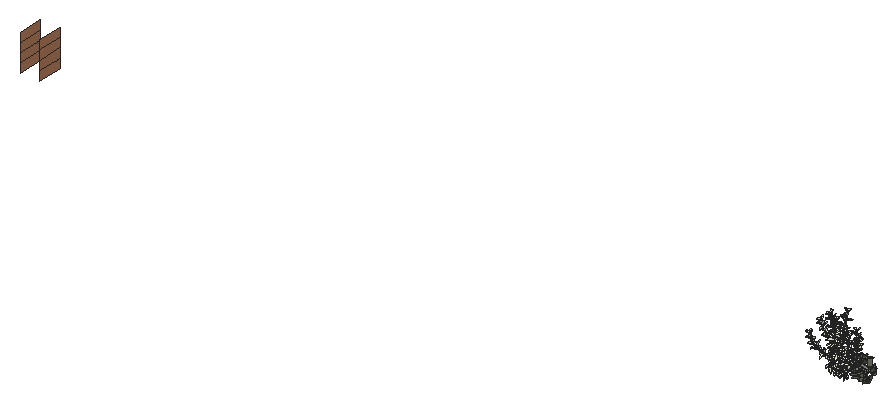
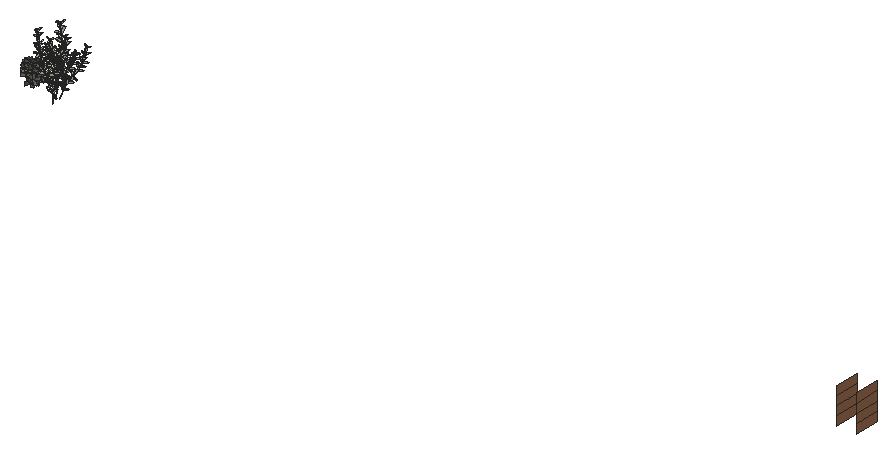
# SketchUp Ruby script. Lengths in inches.
U = 1.inch
M = Sketchup.active_model
def pt(a) = Geom::Point3d.new(a.map { |v| v * U })
def face(e, loops, mat)
  f = e.add_face(loops[0].map { |a| pt(a) })
  loops[1..].each { |l| e.add_face(l.map { |a| pt(a) }).erase! }
  f.material = f.back_material = mat if mat
  f
end
# faces: each face lists its corners as indices into pts; further lists are holes
def faces(e, pts, list, mat = nil) = list.each { |f| face(e, (f[0].is_a?(Array) ? f : [f]).map { |l| l.map { |i| pts[i] } }, mat) }
# xy, xz, yz: faces in a plane at the given z, y or x. An outline is a flat list of corners, or four numbers for a rectangle; further outlines are holes
def ring(l) = l.size == 4 ? [[l[0], l[1]], [l[2], l[1]], [l[2], l[3]], [l[0], l[3]]] : l.each_slice(2).to_a
def flat(e, list, mat, &to3) = list.each { |f| face(e, (f[0].is_a?(Array) ? f : [f]).map { |l| ring(l).map { |u, v| to3.(u, v) } }, mat) }
def xy(e, z, list, mat = nil) = flat(e, list, mat) { |x, y| [x, y, z] }
def xz(e, y, list, mat = nil) = flat(e, list, mat) { |x, z| [x, y, z] }
def yz(e, x, list, mat = nil) = flat(e, list, mat) { |y, z| [x, y, z] }
def lines(e, pts, list) = list.each { |a, b| e.add_line(pt(pts[a]), pt(pts[b])) }
# prism: a flat outline (further loops are holes) pulled along v
def prism(e, loops, v, mat = nil)
  f = face(e, loops, mat); d = Geom::Vector3d.new(v.map { |x| x * U })
  f.pushpull(f.normal.samedirection?(d) ? d.length : -d.length)
end
def box(e, o, s, mat = nil) = prism(e, [[o, [o[0] + s[0], o[1], o[2]], [o[0] + s[0], o[1] + s[1], o[2]], [o[0], o[1] + s[1], o[2]]]], [0, 0, s[2]], mat)
def at(x, y, z, deg = 0) = Geom::Transformation.translation(pt([x, y, z])) * Geom::Transformation.rotation(ORIGIN, Z_AXIS, deg.degrees)
def axes(o, x, y, z) = Geom::Transformation.new([*x, 0, *y, 0, *z, 0, *pt(o).to_a, 1])
def part(name) = M.definitions.add(name)
# library, detail: a bought-in or finely detailed component or shape, given as its bounding box
def library(name, o, s) = part(name).tap { |d| box(d.entities, o, s) }
def detail(e, o, s) = box(e.add_group.entities, o, s)
def put(e, d, t, mat = nil) = e.add_instance(d, t).tap { |i| i.material = mat if mat }
def group(e, t, mat = nil) = e.add_group.tap { |g| g.transformation = t; g.material = mat if mat }.entities
root = M.entities
M.materials.add("0ad16as01f6asdLeafVar1sfd015as60f1as6").color = [231, 235, 211]
M.materials.add("[Tile Ceramic Multi]").color = [165, 115, 84]
M.materials.add("asdfasdf0165f6asdLeafVar1sfd015as60f1as6").color = [231, 235, 211]
M.materials.add("dw_stemssadfasdfa0sdf1s01d6w1").color = [90, 97, 50]
M.materials.add("viburnumblaasdfas0df1w06d").color = [98, 102, 84]
M.materials.add("viburnumbladsadfasdfad0w122").color = [125, 129, 119]
c1 = part("Component\#315")
p = [[0.25,0,0],[2.05,0.01,0.35],[1.81,4.2,1.66],[0,4.19,1.3125]]
faces(c1.entities,p,[[0,1,2,3]],"viburnumbladsadfasdfad0w122")
c2 = part("viburnumblad2")
put(c2.entities,c1,axes([-19.23,-4.49,-32.18],[83.35428,0,0],[0,79.38502,0],[0,0,83.35428]))
c3 = part("Component\#314")
p = [[0.14,0,0],[2.58,0.05,0.25],[2.44,5.11,2.64],[0,5.05,2.39]]
faces(c3.entities,p,[[0,1,2,3]],"viburnumblaasdfas0df1w06d")
c4 = part("viburnumblad1\#2")
put(c4.entities,c3,axes([-37.25,6.23,19.31],[75.98784,0,0],[0,65.50676,0],[0,0,75.98784]))
c5 = part("vdw_leaf\#1")
p = [[0,0,0],[-2.77,1.61,2.32],[-4.3125,6.1,4.5],[-3.97,13.49,6.09],[-2.47,18.57,6.3],[-0.2,22.73,5.75],
  [2.54,19.66,6.85],[4.3,15.93,7.09],[5.03,7.6,5.43],[3.32,1.76,2.74]]
faces(c5.entities,p,[[0,1,2,3,4,5],[0,5,6,7,8,9]],"0ad16as01f6asdLeafVar1sfd015as60f1as6")
c6 = part("dw_branch_3\#2")
p = [[-10.06,-1.6,62.9],[-0.2,1.54,-0.01],[-10.43,1.54,62.72],[0.18,-1.6,0.17],[-23.75,-21.66,88.91],[-25.7,-20.3,89.55],
  [13.4,11.62,104.56],[13.33,13.52,104.47],[-49.25,-41.87,130.3125],[-50.33,-40.21,130.71],[-4.97,21.13,143.98],[35.61,27.99,178.64],
  [-5.09,23.64,143.96],[35.32,29.14,178.46],[-67.7,-55.38,181.06],[-68.34,-54.45,181.62],[-22.8125,33.9,200.59],[-22.94,35.79,200.41],
  [56.61,36.78,229.75],[56.29,38.09,229.57],[-70.63,-67.46,248.85],[-70.72,-66.33,249.5],[-25.05,43.32,240.75],[-24.98,44.26,240.57]]
faces(c6.entities,p,[[0,1,2],[0,3,1],[4,2,5],[4,0,2],[6,0,2],[6,2,7],[8,4,5],[8,5,9],
  [10,6,7],[11,6,7],[10,7,12],[11,7,13],[14,8,9],[14,9,15],[16,10,12],[16,12,17],
  [18,11,13],[18,13,19],[20,14,15],[20,15,21],[22,16,17],[22,17,23]],"dw_stemssadfasdfa0sdf1s01d6w1")
c7 = part("dw_branch3\#2")
put(c7.entities,c5,axes([-70.33,-63.58,233.32],[-1.00752,0.412,0.78596],[-0.24851,-1.22189,0.32195],[0.83141,0.09817,1.01433]))
put(c7.entities,c5,axes([-66.93,-54.91,182.82],[-0.84976,-0.98359,0.33619],[0.99572,-0.74889,0.32577],[-0.05223,0.46521,1.22907]))
put(c7.entities,c5,axes([-46.12,-39.49,126.35],[1.23843,0.5364,0.23552],[-0.56438,0.94474,0.81599],[0.15707,-0.83465,1.07498]))
put(c7.entities,c5,axes([13.0625,13.13,104.77],[-1.01271,0.69982,-0.26884],[-0.74268,-0.99813,0.19939],[-0.10222,0.31872,1.21473]))
put(c7.entities,c5,axes([-18.87,30.42,186.42],[0.36309,1.06515,-0.56675],[-1.14134,0.49515,0.19939],[0.39128,0.45593,1.10754]))
put(c7.entities,c5,axes([-3.2,4.15,75.77],[-1.04153,0.55414,0.44243],[-0.23365,-1.01045,0.71554],[0.6695,0.50943,0.93801]))
put(c7.entities,c5,axes([23.2,19.41,136.3],[-0.65687,-1.11295,-0.05714],[1.05857,-0.61429,-0.20411],[0.15163,-0.1536,1.24868]))
put(c7.entities,c5,axes([-25.57,35.48,201.32],[-0.64726,0.62827,0.87973],[-0.71635,-1.0172,0.19939],[0.80962,-0.39773,0.87973]))
put(c7.entities,c5,axes([-36.37,-32.14,110.35],[-0.80747,1.09962,0.12544],[-0.83333,-0.50188,-0.96467],[-0.72833,-0.64487,0.96467]))
put(c7.entities,c5,axes([-9.89,26.72,156.79],[0.45529,1.02969,0.56572],[-1.16919,0.33753,0.32662],[0.11537,-0.64297,1.07744]))
put(c7.entities,c5,axes([-26.57,46.1,241.0625],[0.00015,0.80921,0.22536],[-0.83985,0.00446,-0.01542],[-0.01605,-0.22532,0.80906]))
put(c7.entities,c5,axes([-9.2,-2.58,61.06],[-1.10001,-0.40312,0.39014],[0.40883,-1.1116,0.00411],[0.35732,0.13566,1.14763]))
put(c7.entities,c5,axes([-69.91,-63.11,233.93],[1.36249,-0.1432,0],[0.13201,1.25603,0.5309],[-0.05549,-0.52799,1.26295]))
put(c7.entities,c5,axes([32.2,25.46,166.13],[0.06878,-1.29051,-0.05714],[1.22165,0.07415,-0.20411],[0.2113,-0.04403,1.24868]))
put(c7.entities,c5,axes([-5.68,-0.66,44.43],[-0.48448,-1.12287,0.17078],[0.98138,-0.33653,0.57135],[-0.48308,0.36756,1.04626]))
put(c7.entities,c5,axes([43.45,32.81,198.64],[0.5408,1.19584,0.14106],[-0.94242,0.32409,0.86557],[0.74952,-0.45533,0.98656]))
put(c7.entities,c5,axes([12.52,14.14,104.98],[1.02694,0.54888,0.41092],[-0.53566,1.05407,-0.06927],[-0.38969,-0.12321,1.13846]))
put(c7.entities,c5,axes([44.55,32.375,198.73],[-0.65687,-1.11295,-0.05714],[1.05857,-0.61429,-0.20411],[0.15163,-0.1536,1.24868]))
put(c7.entities,c5,axes([-5.67,21.17,141.44],[-1.10726,0.43603,-0.32953],[-0.49537,-1.03435,0.29588],[-0.17521,0.40597,1.12589]))
put(c7.entities,c5,axes([55.69,37.84,229.48],[0.18984,0.96334,0.18958],[-0.71996,0.0053,0.69399],[0.66755,-0.26823,0.69457]))
put(c7.entities,c5,axes([-21.52,36.85,205.2],[0.72606,-0.98817,0.14519],[0.94364,0.7084,0.10251],[-0.16885,0.05176,1.19664]))
put(c7.entities,c5,axes([-68.51,-56.35,196.07],[1.16319,0.72381,0],[-0.66725,1.0723,0.5309],[0.28049,-0.45075,1.26295]))
put(c7.entities,c6,at(0.01,-0.09,-0.02),"dw_stemssadfasdfa0sdf1s01d6w1")
put(c7.entities,c5,axes([-2.49,5.18,75.91],[0.78614,-0.90346,-0.30078],[0.86953,0.79562,-0.11715],[0.28546,-0.14014,1.16705]))
put(c7.entities,c5,axes([-23.125,-16.22,82.25],[0.32175,1.32576,0.12544],[-1.33153,0.31835,0.05068],[0.01989,-0.13382,1.3633]))
put(c7.entities,c5,axes([-23.75,41.99,230.3],[0.85958,-0.87451,0.14519],[0.66531,0.75721,0.62192],[-0.54076,-0.36226,1.01955]))
put(c7.entities,c5,axes([27.07,22.48,149.34],[0.92952,-0.64745,-0.62467],[0.50188,1.074,-0.36637],[0.71693,0.02135,1.04468]))
put(c7.entities,c5,axes([17.66,16.25,119.93],[-0.91649,0.83891,-0.3601],[-0.87434,-0.77966,0.40896],[0.0492,0.54447,1.14321]))
put(c7.entities,c5,axes([-68.37,-54.54,181.63],[0.32047,1.28399,0.35434],[-1.33153,0.31835,0.05068],[-0.03484,-0.35624,1.32241]))
put(c7.entities,c5,axes([-28.98,-27.1,96.48],[-0.8814,-0.35966,-0.98523],[0.75246,-1.11336,-0.26672],[-0.73065,-0.71272,0.91382]))
put(c7.entities,c5,axes([-15.23,28.43,172.72],[-1.21149,0.11898,0.32517],[-0.09739,-1.25259,0.09551],[0.33228,0.0667,1.21356]))
put(c7.entities,c5,axes([-17.5625,31.23,186.85],[-0.49275,-1.12287,0.14519],[0.95014,-0.33653,0.62192],[-0.53717,0.36756,1.01955]))
put(c7.entities,c5,axes([26.7,21.22,149.39],[-1.00104,0.22334,0.83093],[0.36894,-1.0402,0.72406],[0.77731,0.78134,0.72643]))
put(c7.entities,c5,axes([-31.125,-24.87,97.38],[0.75482,-0.86936,0.69068],[-0.00159,0.80023,1.00899],[-1.08766,-0.58016,0.45842]))
put(c7.entities,c5,axes([-71.21,-66.73,248.67],[0.25207,0.96771,0],[-0.8921,0.23237,0.38752],[0.375,-0.09768,0.92186]))
put(c7.entities,c5,axes([-24.11,41.05,229.55],[-1.11612,0.51924,-0.26884],[-0.56394,-1.10897,0.19939],[-0.15444,0.29694,1.21473]))
put(c7.entities,c5,axes([6.75,8.37,91.63],[-0.33418,-1.12287,0.39014],[1.13558,-0.33653,0.00411],[0.10478,0.36756,1.14763]))
put(c7.entities,c5,axes([-26,45.89,241.63],[-0.26986,-0.70824,-0.32129],[0.56818,-0.39091,0.38449],[-0.49365,-0.09775,0.63011]))
put(c7.entities,c5,axes([3.74,17.32,124.35],[0.22441,1.22913,-0.16274],[-1.07812,0.11178,-0.64246],[-0.61228,0.25367,1.07162]))
put(c7.entities,c5,axes([-5.44,22.27,140.88],[1.2203,0.00475,0.31374],[-0.097,1.20386,0.35905],[-0.29841,-0.37189,1.1663]))
put(c7.entities,c5,axes([-13.79,29.35,173.31],[0.83169,-0.90108,0.14519],[0.68877,0.73594,0.62192],[-0.55187,-0.34509,1.01955]))
put(c7.entities,c5,axes([-16.92,-7.26,72.98],[1.30647,0.30378,-0.27886],[0.07026,0.74892,1.14503],[0.40633,-1.10623,0.69861]))
put(c7.entities,c5,axes([4.8,17.55,125.22],[-0.25598,-1.17842,0.26559],[1.01553,-0.08455,0.60363],[-0.56975,0.35087,1.00767]))
put(c7.entities,c5,axes([5.3125,8.35,91.45],[0.00638,1.22913,-0.27714],[-1.16413,0.11178,0.46895],[0.48205,0.25367,1.13617]))
put(c7.entities,c5,axes([38.12,30.57,183.07],[1.12534,0.26182,-0.63833],[-0.46674,1.18829,-0.33545],[0.5081,0.51169,1.10563]))
put(c7.entities,c5,axes([-70.41,-60.38,214.47],[-0.41425,1.30587,0],[-1.20383,-0.38188,0.5309],[0.50605,0.16053,1.26295]))
put(c7.entities,c5,axes([37.03,28.75,180.67],[-1.12533,0.00102,-0.63799],[-0.00113,-1.2408,0],[-0.62497,0.00057,1.10237]))
put(c7.entities,c5,axes([30.71,25.35,165.96],[-0.1364,1.29314,0.22715],[-1.08768,-0.23921,0.70862],[0.73536,-0.11394,1.09026]))
put(c7.entities,c5,axes([-38.05,-30.84,110.67],[-0.31533,-1.27379,-0.2839],[1.018,-0.40311,0.67794],[-0.74394,-0.05723,1.08307]))
put(c7.entities,c5,axes([50.11,34.45,213.36],[-1.05669,0.74401,-0.05714],[-0.616,-0.82138,0.69675],[0.37221,0.60904,1.04705]))
put(c7.entities,c5,axes([-65.32,-58.78,200.07],[-1.14597,-0.19668,-0.6713],[0.21784,-1.26924,0],[-0.64812,-0.11124,1.139]))
put(c7.entities,c5,axes([-53.2,-43.37,143.59],[-0.72817,-1.09167,-0.2839],[0.82127,-0.72411,0.67794],[-0.71934,0.19815,1.08307]))
put(c7.entities,c5,axes([-61.1,-50.25,163.67],[-0.52887,1.19686,-0.30066],[-1.10762,-0.57104,-0.32484],[-0.42634,0.12264,1.23812]))
put(c7.entities,c5,axes([-54.12,-42.96,142.67],[0.32175,1.32576,0.12544],[-1.33153,0.31835,0.05068],[0.01989,-0.13382,1.3633]))
put(c7.entities,c5,axes([22.03,20.08,132.3],[1.17066,0.5058,-0.34078],[-0.35758,1.16671,0.50333],[0.49407,-0.35407,1.17172]))
put(c7.entities,c5,axes([-8.59,26.04,158.21],[-0.49275,-1.12287,0.14519],[0.95014,-0.33653,0.62192],[-0.53717,0.36756,1.01955]))
put(c7.entities,c5,axes([49.92,34.03,213.7],[1.24742,-0.35176,0.25024],[0.42127,1.159,-0.4708],[-0.09426,0.52477,1.20753]))
put(c7.entities,c5,axes([-70.34,-67.02,249.05],[-0.57048,-0.79684,0],[0.73827,-0.52855,0.24329],[-0.20203,0.14464,0.92729]))
put(c7.entities,c5,axes([56.04,36.81,228.63],[0.33451,-0.90845,-0.15237],[0.87636,0.33365,-0.06538],[0.11487,-0.11636,0.94597]))
put(c7.entities,c5,axes([-69.93,-60.58,214.88],[-0.45293,-0.99272,-0.78227],[1.14635,-0.58199,0.07483],[-0.40282,-0.65636,1.06615]))
put(c7.entities,c5,axes([-16.77,-8.59,72.7],[-1.22785,0.11509,0.53076],[-0.24879,-1.22495,-0.30991],[0.46742,-0.38989,1.16587]))
put(c7.entities,c5,axes([18.29,17.18,119.24],[1.19981,-0.45946,0.3029],[0.40159,1.22775,0.27158],[-0.37626,-0.1547,1.25575]))
put(c7.entities,c5,axes([-6.73,-0.68,43.74],[0.05346,1.22913,-0.27201],[-1.22696,0.11178,0.26396],[0.28163,0.25367,1.20164]))
put(c7.entities,c5,axes([-58.57,-48.42,160.98],[0.43385,-1.23789,0.39533],[1.04879,0.57965,0.66404],[-0.76727,0.09236,1.13122]))
put(c7.entities,c5,axes([-23.4,38.49,215.38],[0.06762,1.22913,-0.26884],[-1.23909,0.11178,0.19939],[0.21835,0.25367,1.21473]))
put(c7.entities,c5,axes([-22.21,-16.62,83.17],[-0.72817,-1.09167,-0.2839],[0.82127,-0.72411,0.67794],[-0.71934,0.19815,1.08307]))
put(c7.entities,c5,axes([-45.7,-40.77,126.53],[-1.33715,-0.0713,-0.0976],[0.07167,-1.28508,-0.04314],[-0.09306,-0.0492,1.31098]))
put(c7.entities,c5,axes([-22.39,38.51,216.12],[-0.49275,-1.12287,0.14519],[0.95014,-0.33653,0.62192],[-0.53717,0.36756,1.01955]))
c8 = part("vdw_leaf\#2")
p = [[0,0,0],[-2.77,1.61,2.32],[-4.3125,6.1,4.5],[-3.97,13.49,6.09],[-2.47,18.57,6.3],[-0.2,22.73,5.75],
  [2.54,19.66,6.85],[4.3,15.93,7.09],[5.03,7.6,5.43],[3.32,1.76,2.74]]
faces(c8.entities,p,[[0,1,2,3,4,5],[0,5,6,7,8,9]],"asdfasdf0165f6asdLeafVar1sfd015as60f1as6")
c9 = part("dg_branch_1\#2")
p = [[46.12,1.57,35.62],[46,5.42,35.41],[0.14,1.79,0.05],[0.26,-2.0625,0.27],[74.05,2.99,75.8],[74.11,5.28,75.58],
  [103.46,0.47,94.74],[104.03,2.92,94.84],[81.14,16.92,120.46],[81.2,18.78,120.24],[130.47,-5.6875,130.27],[130.58,-3.66,129.85],
  [80.82,34.4375,191.22],[80.64,35.93,190.9],[148.49,-14.56,203.24],[148.9,-12.8125,203.11],[81.08,37.95,226.93],[81.4,39.1,227.03],
  [157.45,-18.19,250.77],[157.7,-17.01,250.41]]
faces(c9.entities,p,[[0,1,2,3],[4,0,1],[4,1,5],[6,4,5],[6,5,7],[8,4,5],[8,5,9],[10,6,7],
  [10,7,11],[12,8,9],[12,9,13],[14,10,11],[14,11,15],[16,12,13],[16,13,17],[18,14,15],
  [18,15,19]],"dw_stemssadfasdfa0sdf1s01d6w1")
c10 = part("vdw_branch1\#3")
put(c10.entities,c8,axes([120.69,-2.42,117.31],[1.12221,-0.24063,-0.65809],[0.19207,1.24776,-0.12871],[0.65778,0.01392,1.11658]))
put(c10.entities,c8,axes([81,38.9,226.05],[0.7888,-0.58155,0],[0.48308,0.65523,0.47],[-0.28484,-0.38635,0.83138]))
put(c10.entities,c8,axes([78.08,12.69,106.05],[-1.43826,-0.02353,-0.03177],[0.0088,-1.31777,0.57755],[-0.03854,0.57714,1.31741]))
put(c10.entities,c8,axes([130.18,-4.73,130.41],[-0.38031,-1.29044,-0.11242],[1.20662,-0.31032,-0.51987],[0.47109,-0.24694,1.24081]))
put(c10.entities,c8,axes([157.08,-17.89,249.93],[-0.91355,0.40674,0],[-0.37496,-0.84216,0.38752],[0.15762,0.35401,0.92186]))
put(c10.entities,c8,axes([90.64,3.03,86.49],[0.32514,-0.85045,-0.99675],[0.69523,0.98247,-0.61148],[1.11061,-0.36604,0.67459]))
put(c10.entities,c8,axes([80.15,28.42,160.95],[-0.16039,0.95636,-1.06292],[-1.41646,0.03966,0.24943],[0.19509,1.07422,0.93709]))
put(c10.entities,c8,axes([126.74,-5.45,129.22],[-0.59819,0.96152,-0.6841],[-0.85772,0.12575,0.92675],[0.75427,0.88089,0.57856]))
put(c10.entities,c8,axes([133.22,-6.12,150.66],[-0.93823,0.76985,0.59124],[-0.47726,-1.08188,0.65135],[0.84525,0.24366,1.02405]))
put(c10.entities,c8,axes([80.43,22.89,141.32],[-1.42571,-0.19312,0.01373],[0.18338,-1.31425,0.5561],[-0.0621,0.5528,1.32692]))
put(c10.entities,c8,axes([33.14,0.88,26.42],[-0.13338,1.31536,0.04876],[-1.04528,-0.13221,0.7073],[0.72315,0.03348,1.07497]))
put(c10.entities,c8,axes([152.63,-15.08,221.76],[-1.28188,0.41945,0.0579],[-0.3638,-1.18547,0.53367],[0.21665,0.49113,1.23869]))
put(c10.entities,c8,axes([80.05,28.28,160.33],[-0.46732,-1.26661,0.40679],[1.27397,-0.40257,0.21004],[-0.07408,0.44645,1.30501]))
put(c10.entities,c8,axes([153.95,-14.8,235.875],[0.39005,1.07743,0.20605],[-0.96443,0.25296,0.50293],[0.42961,-0.3464,0.99807]))
put(c10.entities,c8,axes([80.2,24.22,141.74],[1.33062,-0.46576,0.02628],[0.44746,1.2746,-0.06608],[-0.00197,0.0722,1.37936]))
put(c10.entities,c8,axes([145.48,-12.5,188.92],[-1.32952,0.16983,0.16138],[-0.09299,-1.2361,0.53471],[0.21503,0.51548,1.22904]))
put(c10.entities,c8,axes([139.64,-9.18,171.24],[0.05682,1.30088,0.23414],[-1.13176,-0.05343,0.57151],[0.58357,-0.22963,1.13417]))
put(c10.entities,c8,axes([70.95,4.35,71.98],[-1.1081,-0.41873,0.64752],[0.33675,-1.28259,-0.25313],[0.6937,-0.04625,1.15721]))
put(c10.entities,c8,axes([59.85,4.55,56.17],[-0.26797,1.24526,0.35754],[-0.9369,-0.41634,0.74783],[0.83377,-0.10389,0.98674]))
put(c10.entities,c8,axes([33.11,3.36,25.66],[-0.57817,-1.07968,-0.5679],[1.11554,-0.21356,-0.7297],[0.49375,-0.78178,0.98363]))
put(c10.entities,c9,at(-0.21,0.34,-0.17),"dw_stemssadfasdfa0sdf1s01d6w1")
put(c10.entities,c8,axes([80.91,19.01,122.53],[-0.84258,1.13222,-0.27981],[-1.15093,-0.75138,0.42537],[0.18861,0.47293,1.3457]))
put(c10.entities,c8,axes([119.8,-1.22,114.1],[-1.3235,-0.25012,0.09101],[0.25933,-1.31572,0.15537],[0.05991,0.1698,1.33794]))
put(c10.entities,c8,axes([46.29,5.1,38.04],[0.98937,0.73827,-0.47585],[-0.72359,1.03721,0.10473],[0.44068,0.18581,1.20453]))
put(c10.entities,c8,axes([81.1875,33.03,184.45],[1.33883,0.26986,0.35053],[-0.09581,1.22087,-0.57399],[-0.42216,0.53228,1.20262]))
put(c10.entities,c8,axes([80.16,36.28,206.98],[-0.83993,0.85737,-0.6234],[-1.05964,-0.65701,0.5241],[0.02941,0.81391,1.07976]))
put(c10.entities,c8,axes([154.86,-16.15,234.87],[0.02509,-1.15302,-0.28506],[1.1487,-0.04894,0.29908],[-0.30202,-0.28195,1.11384]))
put(c10.entities,c8,axes([108.77,-0.33,101.14],[-0.47691,-1.03266,-0.72709],[1.25395,-0.29455,-0.40416],[0.15052,-0.81814,1.06325]))
put(c10.entities,c8,axes([89.79,3.01,85.87],[-0.61344,0.75518,0.8965],[-0.17758,-1.01824,0.73622],[1.13385,0.22574,0.58569]))
put(c10.entities,c8,axes([81.56,20.31,123.29],[0.37259,-1.3435,0.21057],[1.29385,0.32364,-0.22445],[0.16906,0.25791,1.34638]))
put(c10.entities,c8,axes([46.45,1.82,36.74],[-0.77883,0.29892,1.0614],[0.19124,-1.24314,0.49044],[1.08598,0.43329,0.67484]))
put(c10.entities,c8,axes([71.37,4.02,72.32],[0.72905,0.81546,-0.74421],[-0.66805,0.98958,0.42988],[0.8391,0.14186,0.97745]))
put(c10.entities,c8,axes([136.59,-5.88,150.53],[0.85845,-0.99897,-0.12437],[0.96526,0.81273,0.13453],[-0.02572,-0.18182,1.28292]))
put(c10.entities,c8,axes([80.375,38.8,225.86],[-0.25178,0.96778,0],[-0.89216,-0.23211,0.38752],[0.37503,0.09757,0.92186]))
put(c10.entities,c8,axes([74.43,7.99,85.38],[-1.05703,0.91669,-0.33543],[-0.95806,-0.87958,0.61531],[0.18697,0.6754,1.25659]))
put(c10.entities,c8,axes([76.57,9.74,89.32],[0.63146,-1.21538,0.33508],[1.18148,0.49387,-0.43517],[0.26321,0.48577,1.26593]))
put(c10.entities,c8,axes([81.6875,36.97,207.4],[0.09422,-1.04424,0.38486],[1.01646,0.1939,0.27727],[-0.33299,0.33382,0.98727]))
put(c10.entities,c8,axes([157.29,-17.17,249.98],[0.50586,-0.50586,0],[0.38853,0.38853,0.41105],[-0.29684,-0.29684,0.56115]))
put(c10.entities,c8,axes([79.92,15.8,106.09],[1.03917,-0.29343,-0.90675],[-0.14587,1.22131,-0.5624],[0.92163,0.5191,0.88824]))
put(c10.entities,c8,axes([61.95,3.88,56.26],[0.41243,-1.28546,0],[1.17466,0.37688,-0.54831],[0.5221,0.16751,1.23363]))
put(c10.entities,c8,axes([151.99,-14.79,208.15],[-0.48571,-1.21723,-0.32393],[1.25386,-0.50033,0],[-0.12005,-0.30087,1.31056]))
put(c10.entities,c8,axes([108.44,0.62,102.22],[0.82183,0.96078,0.38967],[-0.62327,0.08618,1.10203],[0.79141,-0.88661,0.51693]))
put(c10.entities,c8,axes([145.6,-10.56,188.62],[1.03241,-0.02554,-0.82693],[0.3944,1.11584,0.45794],[0.70325,-0.61672,0.89706]))
put(c10.entities,c8,axes([78.59,32.3,183.89],[-1.12675,-0.42036,0.43987],[0.5899,-0.98149,0.57312],[0.14901,0.70693,1.05726]))
put(c10.entities,c8,axes([152.08,-13.42,223.37],[0.79993,-0.44251,-0.69938],[0.68456,0.82615,0.26026],[0.41048,-0.60953,0.85515]))
put(c10.entities,c8,axes([140.71,-8.74,170.55],[0.41903,-1.24177,-0.32393],[1.26224,0.33728,0.33986],[-0.23168,-0.40836,1.26573]))
put(c10.entities,c8,axes([149.25,-12.53,205.78],[1.24456,0.38285,0.23414],[-0.42999,1.04826,0.57151],[-0.02056,-0.62679,1.13417]))
yz(root,1457.08,[[340.22,0,362.07,8],[340.22,8,362.07,16],[340.22,16,362.07,24],[340.22,24,362.07,32]],"[Tile Ceramic Multi]")
yz(root,1474.64,[[340.22,0,362.07,8],[340.22,8,362.07,16],[340.22,16,362.07,24],[340.22,24,362.07,32]],"[Tile Ceramic Multi]")
put(root,c2,axes([2203.77,343.25,21.47],[-0.00563,0.00838,0.00295],[-0.00922,-0.00664,0.00128],[0.00288,-0.0019,0.0109]))
put(root,c4,axes([2203.71,345.64,16.93],[-0.01133,-0.00353,0.00405],[0.00312,-0.01382,-0.0033],[0.00465,-0.0017,0.01152]))
put(root,c4,axes([2195.84,342.28,24.87],[-0.00055,0.01258,-0.0057],[-0.01484,-0.00329,-0.00573],[-0.0051,0.00524,0.0099]))
put(root,c4,axes([2202.68,345.08,14.41],[-0.00681,0.00895,0.00759],[-0.01184,-0.01026,0.00148],[0.00579,-0.00507,0.01117]))
put(root,c2,axes([2204.95,342.48,26.28],[0,0.01516,0.00154],[-0.01516,-0.00015,0.00148],[0.00149,-0.00153,0.01509]))
put(root,c2,axes([2197.1875,344.04,21.98],[0.00305,-0.01398,-0.00068],[0.01153,0.00223,0.00588],[-0.00601,-0.00193,0.01207]))
put(root,c7,axes([2176.85,351.625,3.93],[-0.08978,-0.1003,-0.04713],[0.10044,-0.06083,-0.0937],[0.03793,-0.07633,0.13659]))
put(root,c2,axes([2203.21,342.7,22.78],[0.00269,0.01067,0.0031],[-0.01059,0.00139,0.00439],[0.00368,-0.00386,0.01011]))
put(root,c4,axes([2201.96,345.83,12.97],[-0.00857,-0.01458,-0.00131],[0.01562,-0.00975,0.00697],[-0.00558,0.00226,0.01502]))
put(root,c2,axes([2196.07,341.64,23.18],[0.00718,0.01175,0.00394],[-0.01195,0.00776,-0.0014],[-0.003,-0.00258,0.01303]))
put(root,c4,axes([2195.77,344.53,26.35],[-0.01073,0.0028,-0.00658],[-0.00691,-0.01149,0.00571],[-0.00344,0.00773,0.00806]))
put(root,c2,axes([2197.59,342.11,20.14],[0.00689,0.01128,0.00378],[-0.0129,0.00838,-0.00151],[-0.003,-0.00258,0.01303]))
put(root,c2,axes([2193.89,345.8125,17.95],[-0.00567,0.00572,-0.00867],[-0.00649,-0.01145,-0.00331],[-0.00924,0.00313,0.00728]))
put(root,c2,axes([2202.95,342.875,24.48],[0.00958,0.00624,0.00001],[-0.00544,0.00834,0.00562],[0.00306,-0.00472,0.00995]))
put(root,c2,axes([2192.88,346.62,18.95],[-0.0076,-0.00349,-0.00917],[-0.00045,-0.01161,0.00442],[-0.00992,0.00325,0.00636]))
put(root,c2,axes([2195.97,343.4375,23.375],[0.01149,-0.00801,0.00297],[0.00658,0.01147,0.00547],[-0.00527,-0.00304,0.01219]))
put(root,c2,axes([2191.42,345.89,19.77],[-0.00591,0.00596,-0.00904],[-0.00601,-0.0106,-0.00307],[-0.00924,0.00313,0.00728]))
put(root,c2,axes([2197.32,343.91,20.32],[0.012,-0.00837,0.00311],[0.00592,0.01032,0.00492],[-0.00527,-0.00304,0.01219]))
put(root,c2,axes([2196.44,342.59,21.5625],[0.0132,0.00264,0.00489],[-0.00375,0.01436,0.00234],[-0.00402,-0.00331,0.01259]))
put(root,c2,axes([2202.67,343.9375,23.34],[0.01085,-0.00184,-0.00308],[0.00296,0.01015,0.00436],[0.00203,-0.00494,0.01011]))
put(root,c4,axes([2195.67,344.72,15.49],[-0.00086,0.01375,0.00031],[-0.0113,-0.00049,-0.01107],[-0.00962,-0.00074,0.00907]))
put(root,c2,axes([2204.29,343.13,24.39],[0.01077,0.01069,0.00135],[-0.01074,0.01048,0.00267],[0.00094,-0.00284,0.01494]))
put(root,c4,axes([2200.22,346.37,20.91],[-0.01012,-0.01025,0.00891],[0.01634,-0.00922,0.0075],[0.00063,0.01164,0.0125]))
put(root,c2,axes([2199.56,347.66,21.55],[-0.01264,0.00008,-0.0032],[-0.00094,-0.01268,0.00342],[-0.00306,0.00351,0.01217]))
put(root,c2,axes([2192.3,345.45,18.41],[-0.00076,0.01192,-0.00361],[-0.00919,-0.00341,-0.00868],[-0.0089,0.00223,0.00792]))
put(root,c7,axes([2170.38,352.45,10.58],[0.11088,0.06382,0.04174],[-0.06957,0.11109,0.02262],[-0.01961,-0.03323,0.15579]))
put(root,c4,axes([2202.19,347.72,11.95],[-0.01097,-0.01069,0.00215],[0.01213,-0.01096,0.00739],[-0.00308,0.00597,0.01392]))
put(root,c2,axes([2191.49,347.45,19.52],[-0.00484,-0.0109,-0.00393],[0.00466,-0.0057,0.0098],[-0.01055,0.00253,0.0057]))
put(root,c4,axes([2194.68,346.55,26.76],[-0.01129,-0.00613,-0.00067],[0.00417,-0.00777,0.01127],[-0.0047,0.00912,0.00614]))
put(root,c4,axes([2198.06,343.74,16.89],[0.01357,-0.0015,0.0077],[-0.00069,0.01762,0.00453],[-0.00774,-0.0037,0.01228]))
put(root,c4,axes([2199.32,345.42,15.01],[0.00765,-0.01303,0.00422],[0.01267,0.01016,0.00822],[-0.00817,-0.00039,0.01254]))
put(root,c2,axes([2198.5,347.08,23.1],[-0.00854,0.00917,-0.00359],[-0.00964,-0.00875,0.0006],[-0.00199,0.00305,0.01252]))
put(root,c2,axes([2193.14,347.59,28.69],[-0.01044,-0.00252,-0.00593],[-0.00181,-0.00803,0.006],[-0.00557,0.00722,0.00577]))
put(root,c2,axes([2199.63,348.34,19.93],[-0.00812,-0.00859,-0.00204],[0.0081,-0.00886,0.00508],[-0.00515,0.00206,0.01179]))
put(root,c7,axes([2176.64,348.96,7.47],[0.05022,0.15549,0],[-0.15549,0.05022,0],[0,0,0.20106]))
put(root,c2,axes([2198.85,348.68,22.94],[-0.00933,-0.00906,-0.00093],[0.0081,-0.00886,0.00508],[-0.00417,0.00306,0.01196]))
put(root,c2,axes([2205.48,345.93,26.37],[0.00259,0.01229,-0.00001],[-0.01185,0.00249,-0.00335],[-0.00327,0.0007,0.01211]))
put(root,c2,axes([2192.88,345.5,16.77],[0.00505,0.01138,0.0041],[-0.00637,0.00552,-0.00732],[-0.00911,0.00107,0.00791]))
put(root,c4,axes([2204.73,344.07,28.21],[0.00918,0.0099,-0.00625],[-0.01245,0.01197,0.0007],[0.0045,0.00408,0.01216]))
put(root,c4,axes([2196.67,344.78,13.27],[0.00499,0.00892,0.00903],[-0.00667,0.01209,-0.00778],[-0.01141,-0.0013,0.00685]))
put(root,c2,axes([2192.16,346.79,28.65],[0.00165,0.00828,-0.00613],[-0.01063,-0.00165,-0.00484],[-0.00434,0.00735,0.00651]))
put(root,c2,axes([2192.22,347.59,17.875],[0.00076,-0.01192,0.00361],[0.0064,0.00373,0.01004],[-0.01075,0.00137,0.00569]))
put(root,c2,axes([2190.46,345.72,18.55],[0.00484,0.0109,0.00393],[-0.00707,0.00614,-0.00813],[-0.00911,0.00107,0.00791]))
put(root,c2,axes([2198.22,346.69,21.37],[0.00055,0.01289,-0.00188],[-0.01292,0.00032,-0.00165],[-0.00158,0.00193,0.01279]))
put(root,c10,axes([2176.29,348.59,7.1875],[0.13835,-0.02464,0],[0.02464,0.13835,0],[0,0,0.17291]))
put(root,c4,axes([2197.38,347.82,24.14],[-0.00372,0.0118,-0.00306],[-0.01362,-0.00502,-0.00283],[-0.00309,0.00191,0.01102]))
put(root,c4,axes([2198.25,349.27,25.21],[-0.00969,-0.0086,0.00402],[0.01095,-0.00941,0.00625],[-0.00101,0.00665,0.01178]))
put(root,c4,axes([2197.29,349.53,25.9],[-0.0112,0.0013,-0.00343],[-0.00292,-0.0124,0.00476],[-0.00244,0.00473,0.0094]))
put(root,c2,axes([2191.57,346.04,17.3],[0.0076,0.00349,0.00917],[-0.0018,0.01107,-0.00252],[-0.00973,0.00035,0.00724]))
put(root,c2,axes([2198.37,348.95,21.01],[-0.00055,-0.01289,0.00188],[0.01116,0.00015,0.00431],[-0.00466,0.00195,0.01201]))
put(root,c2,axes([2192.82,346.84,16.5625],[0.00644,-0.0055,0.00764],[0.00359,0.01104,0.00474],[-0.00972,-0.00018,0.00726]))
put(root,c2,axes([2192.46,348.32,27.63],[-0.00127,-0.00935,0.00568],[0.00996,0.00338,0.00695],[-0.00695,0.00574,0.0058]))
put(root,c4,axes([2198.77,345.98,11.5625],[0.00484,-0.00571,0.01239],[0.00394,0.01587,0.00555],[-0.01361,0.00143,0.00513]))
put(root,c2,axes([2190.53,347.28,18.3],[0.00591,-0.00596,0.00904],[0.00359,0.01104,0.00474],[-0.01042,0.00047,0.00632]))
put(root,c2,axes([2190.73,348.3125,30.14],[0.00132,0.00974,-0.00592],[-0.01063,-0.00165,-0.00484],[-0.00451,0.00633,0.00719]))
put(root,c2,axes([2198.12,346.86,19.63],[0.00895,0.00869,0.00089],[-0.00957,0.01008,-0.0022],[-0.00208,0.00083,0.01284]))
put(root,c2,axes([2198.32,348.5,19.47],[0.00892,-0.00957,0.00375],[0.00799,0.0083,0.0022],[-0.00426,0.00084,0.01229]))
put(root,c4,axes([2199.96,348.37,14.1],[0.00413,-0.01232,0.00597],[0.01417,0.00711,0.00487],[-0.00618,0.00389,0.01229]))
put(root,c4,axes([2201.47,350.01,19.36],[-0.01045,-0.00476,0.01095],[0.01292,-0.01059,0.00773],[0.00429,0.01208,0.00936]))
put(root,c2,axes([2190.88,347.61,28.82],[0.008,0.00859,-0.00017],[-0.00687,0.00594,-0.00742],[-0.00498,0.00541,0.0075]))
put(root,c2,axes([2196.94,347.37,22.66],[0.00933,0.00906,0.00093],[-0.00886,0.00934,-0.00204],[-0.00208,0.00083,0.01284]))
put(root,c2,axes([2195.52,350.56,17.12],[-0.00445,0.00477,-0.00883],[-0.0086,-0.00885,-0.00045],[-0.00678,0.00624,0.00678]))
put(root,c4,axes([2197.04,348.27,24.12],[0.00188,0.00994,-0.00772],[-0.0143,-0.00023,-0.00375],[-0.00243,0.00751,0.00854]))
put(root,c4,axes([2198.46,347.93,23.44],[0.00743,-0.01098,0.00888],[0.01612,0.00899,-0.00172],[-0.00302,0.0089,0.01251]))
put(root,c2,axes([2197.29,348.97,22.5],[0.00854,-0.00917,0.00359],[0.00887,0.00923,0.00245],[-0.00426,0.00084,0.01229]))
put(root,c4,axes([2196.11,351,26.82],[-0.00897,-0.00759,0.00065],[0.00732,-0.00776,0.00825],[-0.00418,0.00599,0.00812]))
put(root,c4,axes([2196.62,348.74,14.92],[0.0024,0.01209,-0.00232],[-0.01101,0.00036,-0.0095],[-0.00784,0.00332,0.00921]))
put(root,c2,axes([2197.35,347.8,20.94],[0.01264,-0.00008,0.0032],[0.00017,0.01368,-0.00036],[-0.00319,0.00037,0.01263]))
put(root,c2,axes([2191.23,348.9,28.18],[0.00614,-0.00518,0.0082],[0.00724,0.00927,0.00063],[-0.0067,0.00499,0.00652]))
put(root,c2,axes([2194.9,351.68,17.95],[-0.00828,-0.00278,-0.00738],[-0.00265,-0.00909,0.0064],[-0.00743,0.00635,0.00594]))
put(root,c4,axes([2198.62,347.57,16.26],[0.01227,-0.00323,0.0066],[0.00379,0.01612,0.00085],[-0.00658,0.00088,0.01266]))
put(root,c2,axes([2205.34,351.03,23.19],[-0.00964,0.00707,-0.00598],[-0.00922,-0.00808,0.00531],[-0.0008,0.00796,0.01071]))
put(root,c4,axes([2197.62,350.48,25.08],[-0.00938,0.00386,-0.00599],[-0.00819,-0.00718,0.008],[-0.00057,0.00892,0.00623]))
put(root,c2,axes([2194.3,350.375,29.12],[-0.00122,0.00857,-0.00461],[-0.01002,-0.00286,-0.00259],[-0.0035,0.00446,0.00809]))
put(root,c2,axes([2193.53,351.55,18.95],[-0.00463,0.00496,-0.0092],[-0.00796,-0.0082,-0.00042],[-0.00678,0.00624,0.00678]))
put(root,c4,axes([2197.33,348.16,12.77],[0.00721,0.00805,0.00636],[-0.00379,0.01064,-0.00917],[-0.00973,0.00288,0.00737]))
put(root,c2,axes([2198.4,348.4375,29.91],[0.00912,0.00933,-0.00467],[-0.01186,0.01016,-0.00285],[0.00181,0.00573,0.01291]))
put(root,c2,axes([2204.9,350.05,21.77],[-0.00039,0.0109,-0.00675],[-0.01442,-0.00054,-0.00004],[-0.00029,0.00703,0.01137]))
put(root,c4,axes([2196.55,350.14,27.23],[0.00379,-0.01036,0.00596],[0.01309,0.006,0.00209],[-0.00395,0.00482,0.01088]))
put(root,c4,axes([2199.29,348.375,10.8125],[0.00403,-0.00389,0.01235],[0.00756,0.01368,0.00184],[-0.01119,0.00546,0.00538]))
put(root,c2,axes([2190.14,349.14,29.11],[0.01,0.00241,0.00568],[0.00061,0.01041,-0.00507],[-0.00589,0.00485,0.00722]))
put(root,c2,axes([2194.08,350.71,17.71],[0.00173,0.0098,-0.00563],[-0.00961,-0.00223,-0.00684],[-0.00663,0.00549,0.00752]))
put(root,c2,axes([2198.41,350.11,29.13],[0.01161,-0.00902,0.00438],[0.00853,0.00943,-0.00297],[-0.0007,0.0056,0.01299]))
put(root,c4,axes([2197.79,347.92,26.21],[0.01555,-0.00131,0.00405],[0.00291,0.01735,-0.00577],[-0.00307,0.00585,0.01401]))
put(root,c2,axes([2193.92,352.83,18.41],[-0.00707,-0.00889,-0.00124],[0.00366,-0.00429,0.00994],[-0.0082,0.00576,0.0055]))
put(root,c2,axes([2194.46,350.33,16.14],[0.00739,0.00929,0.00129],[-0.00498,0.005,-0.00749],[-0.00707,0.00455,0.00775]))
put(root,c4,axes([2204.25,348.75,18.51],[0.01166,0.00889,0.00003],[-0.00952,0.01251,-0.00648],[-0.00341,0.00442,0.01356]))
put(root,c2,axes([2194.1,351.94,28.37],[0.00162,-0.00936,0.00394],[0.00963,0.00389,0.00496],[-0.00566,0.00263,0.0077]))
put(root,c2,axes([2193.09,350.8,29.67],[0.00555,0.00919,-0.00035],[-0.00852,0.00498,-0.00446],[-0.00353,0.00247,0.00881]))
put(root,c2,axes([2204.13,351.51,24.71],[-0.00041,0.01136,-0.00703],[-0.01336,-0.0005,-0.00003],[-0.00029,0.00703,0.01137]))
put(root,c2,axes([2194.46,352.47,16.81],[-0.00173,-0.0098,0.00563],[0.00735,0.00343,0.00822],[-0.00865,0.00481,0.00572]))
put(root,c4,axes([2197.16,352.56,25.13],[-0.01138,-0.00264,0.00129],[0.00289,-0.0057,0.01174],[-0.00153,0.01008,0.00426]))
put(root,c2,axes([2194.7,351.45,15.69],[0.00508,-0.00494,0.00777],[0.00608,0.00946,0.00204],[-0.00795,0.00351,0.00743]))
put(root,c2,axes([2192.54,351.42,17.91],[0.00707,0.00889,0.00124],[-0.00553,0.00556,-0.00832],[-0.00707,0.00455,0.00775]))
put(root,c2,axes([2193.48,351.2,16.61],[0.00828,0.00278,0.00738],[0.00071,0.00951,-0.00438],[-0.00785,0.00396,0.00731]))
put(root,c2,axes([2203.85,350.97,22.94],[0.00906,0.00899,-0.00397],[-0.01029,0.00825,-0.00478],[-0.00073,0.006,0.01192]))
